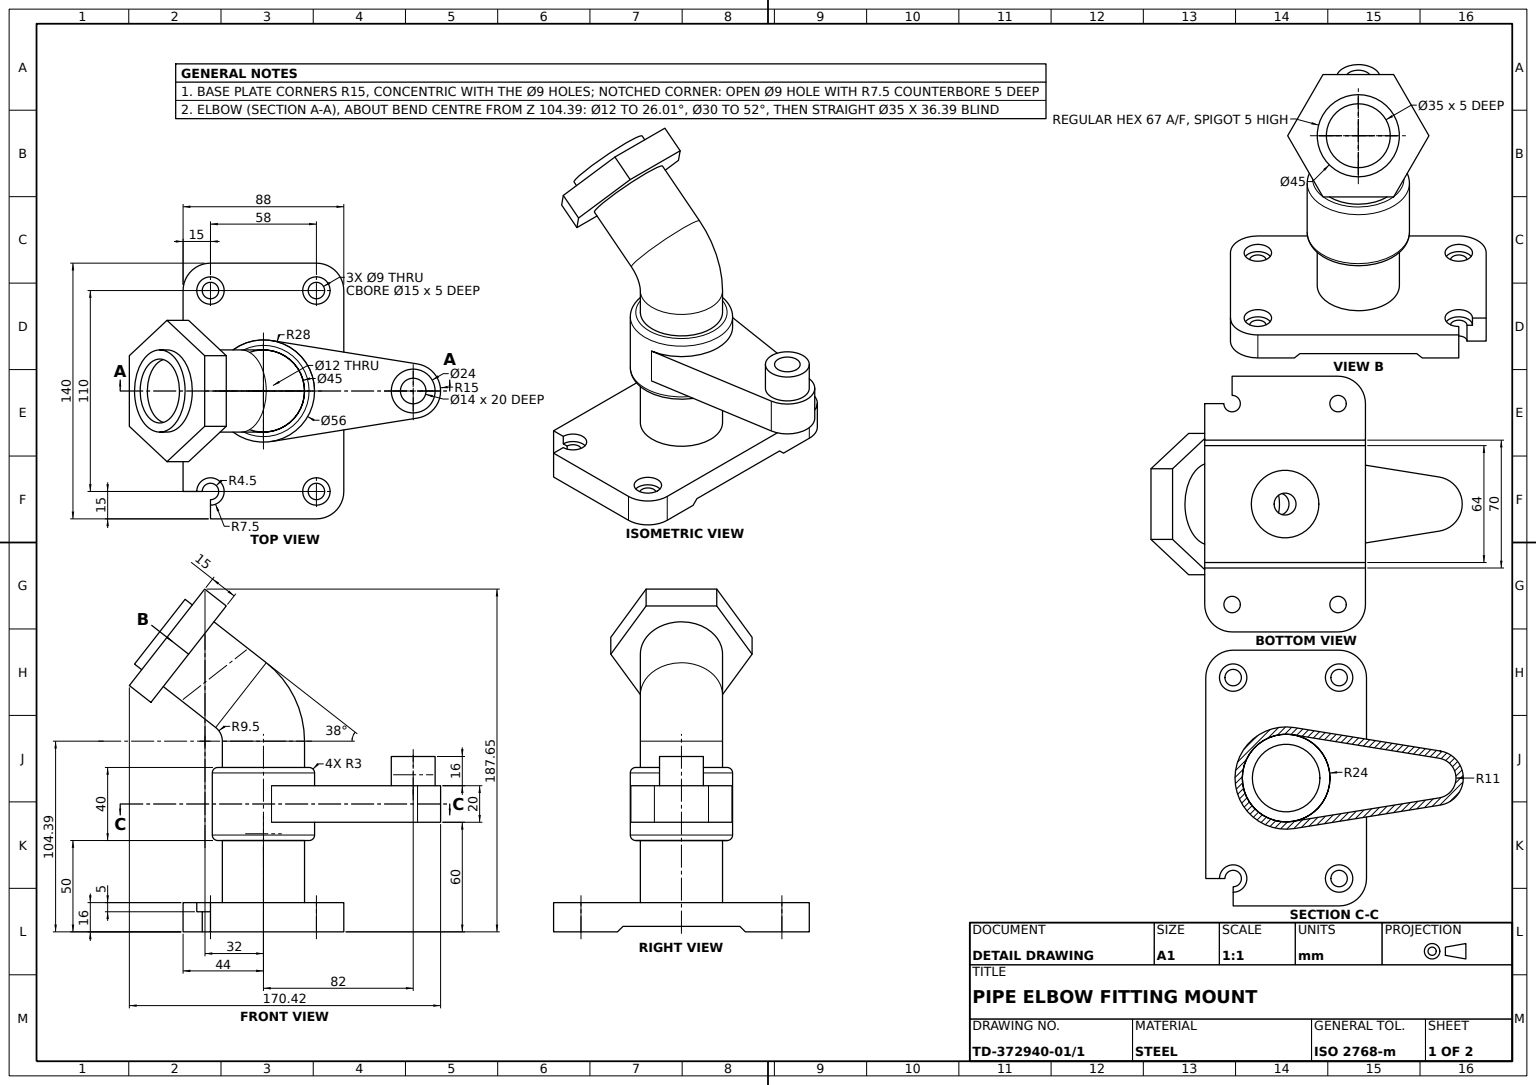
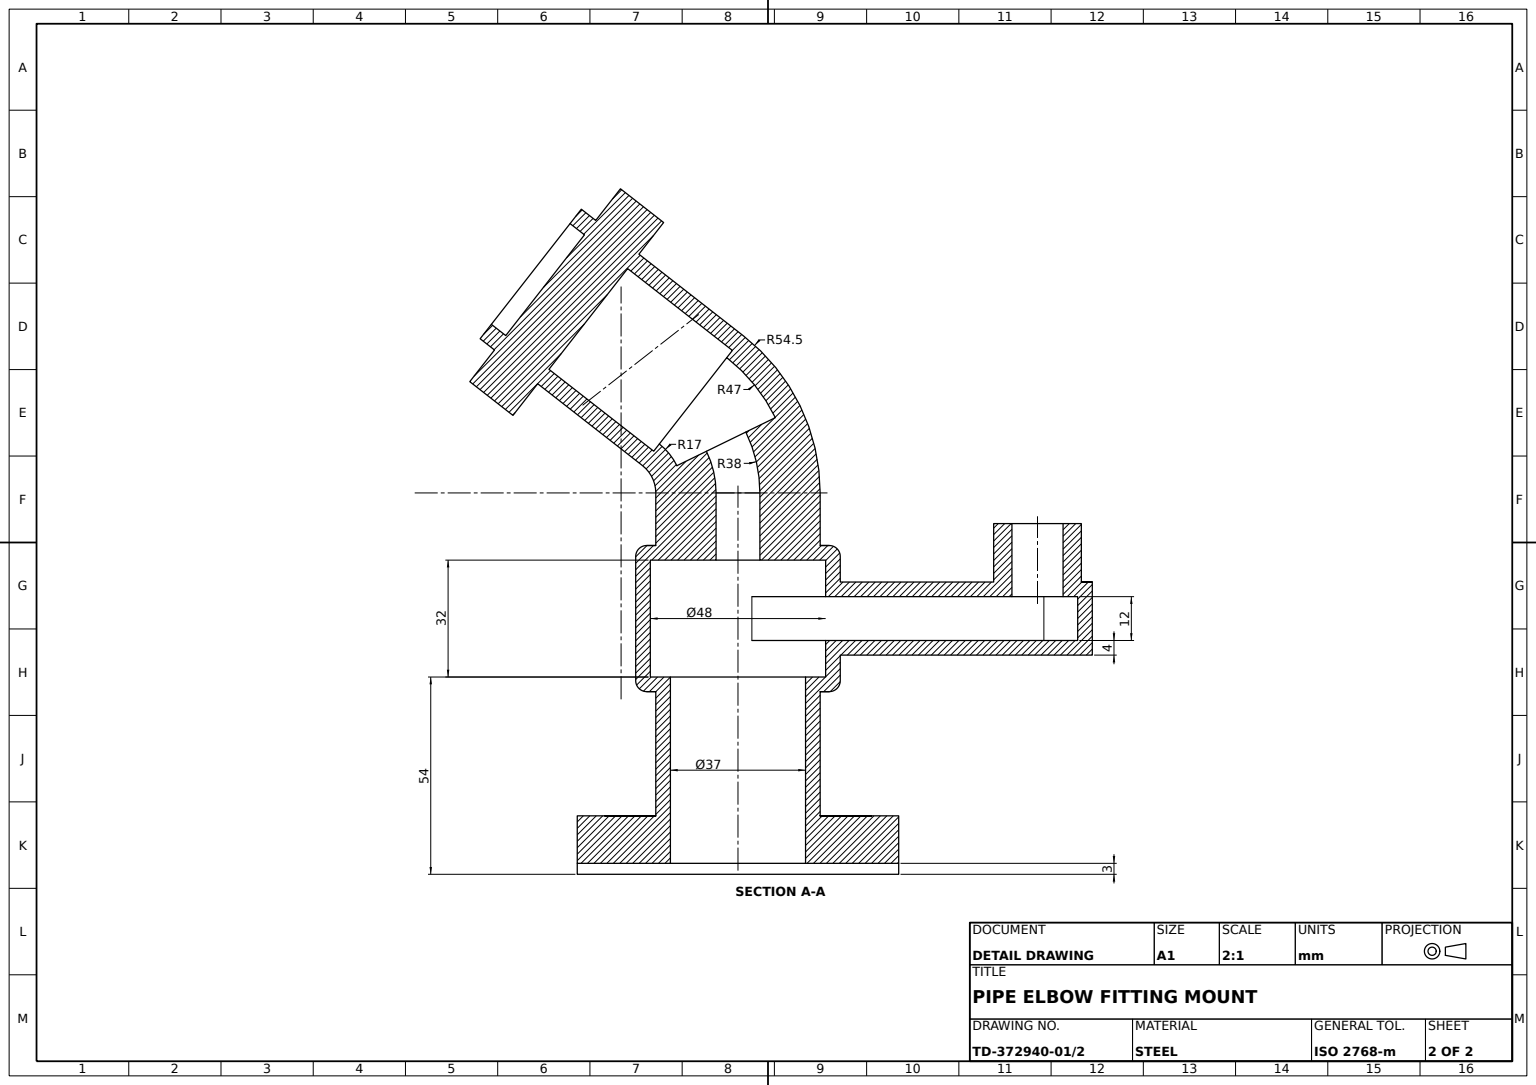
solid
v1 (23.696474,64,-3.804878)
v2 (10.860884,64,-83.743902)
e1 v1 v2 LINE
v3 (-10.860884,64,-83.743902)
e2 v2 v3 CIRCLE(AX(P(0,64,-82),D(0,1,0),D(0,0,1)),11)
v4 (-23.696474,64,-3.804878)
e3 v3 v4 LINE
v5 (0,64,-24)
e4 v4 v5 CIRCLE(AX(P(0,64,0),D(0,-1,0),D(0,0,1)),24)
e5 v5 v1 CIRCLE(AX(P(0,64,0),D(0,-1,0),D(0,0,1)),24)
face PLANE(AX(P(0,64,-82),D(0,1,0),D(0,0,1))) [e1 e2 e3 e4 e5]
v6 (10.860884,76,-83.743902)
v7 (-10.860884,76,-83.743902)
e6 v6 v7 CIRCLE(AX(P(0,76,-82),D(0,1,0),D(0,0,1)),11)
e7 v3 v7 LINE
e8 v2 v6 LINE
face CYL(AX(P(0,64,-82),D(0,1,0),D(0,0,1)),11) rev [e6 -e7 -e2 e8]
v8 (0,178.117814,45.962698)
v9 (0,150.537438,67.51085)
e9 v8 v9 CIRCLE(AX(P(0,164.327626,56.736774),D(0,0.615661475,0.788010754),D(0,-0.788010754,0.615661475)),17.5)
v10 (0,147.459131,63.570796)
e10 v10 v9 LINE
v11 (0,175.039507,42.022645)
e11 v10 v11 CIRCLE(AX(P(0,161.249319,52.79672),D(0,-0.615661475,-0.788010754),D(0,-0.788010754,0.615661475)),17.5)
e12 v11 v8 LINE
face CYL(AX(P(0,129.608901,12.298833),D(0,0.615661475,0.788010754),D(0,-0.788010754,0.615661475)),17.5) rev [e9 -e10 e11 e12]
v12 (-70,0,-29)
v13 (-55,0,-44)
e13 v12 v13 CIRCLE(AX(P(-55,0,-29),D(0,-1,0),D(0,0,1)),15)
v14 (-70,16,-29)
e14 v14 v12 LINE
v15 (-55,16,-44)
e15 v15 v14 CIRCLE(AX(P(-55,16,-29),D(0,1,0),D(0,0,1)),15)
e16 v13 v15 LINE
face CYL(AX(P(-55,16,-29),D(0,-1,0),D(0,0,-1)),15) [-e13 -e14 -e15 -e16]
v16 (55,11,33.5)
v17 (55,11,36.5)
e17 v16 v17 LINE
v18 (59.5,11,29)
e18 v18 v16 CIRCLE(AX(P(55,11,29),D(0,1,0),D(0,0,1)),4.5)
v19 (62.5,11,29)
e19 v18 v19 LINE
e20 v19 v17 CIRCLE(AX(P(55,11,29),D(0,1,0),D(0,0,1)),7.5)
face PLANE(AX(P(59.5,11,29),D(0,-1,0),D(0,0,-1))) rev [-e17 -e18 e19 e20]
v20 (-70,16,29)
e21 v14 v20 LINE
v21 (-70,0,29)
e22 v12 v21 LINE
e23 v21 v20 LINE
face PLANE(AX(P(-70,16,-44),D(1,0,0),D(0,0,-1))) rev [-e21 e14 e22 e23]
v22 (0,146.597384,70.589157)
v23 (0,182.057868,42.884391)
e24 v22 v23 CIRCLE(AX(P(0,164.327626,56.736774),D(0,-0.615661475,-0.788010754),D(0,0.788010754,-0.615661475)),22.5)
e25 v23 v22 CIRCLE(AX(P(0,164.327626,56.736774),D(0,-0.615661475,-0.788010754),D(0,0.788010754,-0.615661475)),22.5)
e26 v9 v8 CIRCLE(AX(P(0,164.327626,56.736774),D(0,0.615661475,0.788010754),D(0,-0.788010754,0.615661475)),17.5)
face PLANE(AX(P(0,164.327626,56.736774),D(0,-0.615661475,-0.788010754),D(0,0.788010754,-0.615661475))) rev [-e24 -e25] [-e26 -e9]
v24 (0,54,18.5)
v25 (0,54,-18.5)
e27 v24 v25 CIRCLE(AX(P(0,54,0),D(0,-1,0),D(0,0,1)),18.5)
e28 v25 v24 CIRCLE(AX(P(0,54,0),D(0,-1,0),D(0,0,1)),18.5)
v26 (0,54,-24)
v27 (0,54,24)
e29 v26 v27 CIRCLE(AX(P(0,54,0),D(0,-1,0),D(0,0,-1)),24)
e30 v27 v26 CIRCLE(AX(P(0,54,0),D(0,-1,0),D(0,0,-1)),24)
face PLANE(AX(P(0,54,24),D(0,1,0),D(0,0,1))) [e27 e28] [-e29 -e30]
v28 (0,80,-97)
v29 (0,60,-97)
e31 v28 v29 LINE
v30 (14.810297,80,-84.378049)
e32 v30 v28 CIRCLE(AX(P(0,80,-82),D(0,1,0),D(0,0,1)),15)
v31 (14.810297,60,-84.378049)
e33 v30 v31 LINE
e34 v31 v29 CIRCLE(AX(P(0,60,-82),D(0,1,0),D(0,0,1)),15)
face CYL(AX(P(0,80,-82),D(0,-1,0),D(0,0,-1)),15) [-e31 -e32 e33 e34]
v32 (0,141.429063,3.063911)
v33 (0,117.78874,21.533755)
e35 v32 v33 CIRCLE(AX(P(0,129.608901,12.298833),D(0,-0.615661475,-0.788010754),D(0,-0.788010754,0.615661475)),15)
v34 (0,125.002777,-10.240014)
e36 v34 v32 CIRCLE(AX(P(0,104.392557,32),D(1,0,0),D(0,0,-1)),47)
v35 (0,111.847318,16.721697)
e37 v35 v34 CIRCLE(AX(P(0,118.425048,3.240841),D(0,0.898723712,0.438515324),D(0,-0.438515324,0.898723712)),15)
e38 v35 v33 CIRCLE(AX(P(0,104.392557,32),D(1,0,0),D(0,0,-1)),17)
face TORUS(AX(P(0,104.392557,32),D(1,0,0),D(0,0,-1)),32,15) rev [-e35 -e36 -e37 e38]
v36 (-55,0,24.5)
v37 (-55,11,24.5)
e39 v36 v37 LINE
v38 (-55,11,33.5)
e40 v37 v38 CIRCLE(AX(P(-55,11,29),D(0,1,0),D(0,0,1)),4.5)
v39 (-55,0,33.5)
e41 v39 v38 LINE
e42 v36 v39 CIRCLE(AX(P(-55,0,29),D(0,1,0),D(0,0,1)),4.5)
face CYL(AX(P(-55,16,29),D(0,1,0),D(0,0,1)),4.5) rev [e39 e40 -e41 -e42]
e43 v33 v32 CIRCLE(AX(P(0,129.608901,12.298833),D(0,-0.615661475,-0.788010754),D(0,-0.788010754,0.615661475)),15)
e44 v34 v35 CIRCLE(AX(P(0,118.425048,3.240841),D(0,0.898723712,0.438515324),D(0,-0.438515324,0.898723712)),15)
face TORUS(AX(P(0,104.392557,32),D(1,0,0),D(0,0,-1)),32,15) rev [-e43 -e38 -e44 e36]
v40 (0,90,-22.5)
v41 (0,104.392557,-22.5)
e45 v40 v41 LINE
v42 (0,104.392557,22.5)
e46 v41 v42 CIRCLE(AX(P(0,104.392557,0),D(0,-1,0),D(0,0,-1)),22.5)
v43 (0,90,22.5)
e47 v43 v42 LINE
e48 v43 v40 CIRCLE(AX(P(0,90,0),D(0,1,0),D(0,0,1)),22.5)
face CYL(AX(P(0,0,0),D(0,1,0),D(0,0,1)),22.5) [e45 e46 -e47 e48]
v44 (0,3,-18.5)
v45 (0,3,18.5)
e49 v44 v45 CIRCLE(AX(P(0,3,0),D(0,1,0),D(0,0,1)),18.5)
e50 v45 v44 CIRCLE(AX(P(0,3,0),D(0,1,0),D(0,0,1)),18.5)
v46 (32,3,-44)
v47 (32,3,44)
e51 v46 v47 LINE
v48 (-32,3,44)
e52 v47 v48 LINE
v49 (-32,3,-44)
e53 v49 v48 LINE
e54 v49 v46 LINE
face PLANE(AX(P(32,3,-97.001),D(0,1,0),D(0,0,1))) rev [e49 e50] [e51 e52 -e53 e54]
v50 (62.5,16,29)
v51 (70,16,29)
e55 v50 v51 LINE
e56 v19 v50 LINE
v52 (59.5,0,29)
e57 v52 v18 LINE
v53 (70,0,29)
e58 v53 v52 LINE
e59 v51 v53 LINE
face PLANE(AX(P(55,-0.001,29),D(0,0,1),D(1,0,0))) [-e55 -e56 -e19 -e57 -e58 -e59]
e60 v40 v43 CIRCLE(AX(P(0,90,0),D(0,1,0),D(0,0,1)),22.5)
v54 (0,90,25)
v55 (0,90,-25)
e61 v54 v55 CIRCLE(AX(P(0,90,0),D(0,1,0),D(0,0,1)),25)
e62 v55 v54 CIRCLE(AX(P(0,90,0),D(0,1,0),D(0,0,1)),25)
face PLANE(AX(P(0,90,0),D(0,1,0),D(0,0,1))) [-e60 -e48] [e61 e62]
v56 (0,80,-28)
v57 (-27.645887,80,-4.439024)
e63 v56 v57 CIRCLE(AX(P(0,80,0),D(0,1,0),D(0,0,1)),28)
v58 (-27.645887,60,-4.439024)
e64 v57 v58 LINE
v59 (0,60,-28)
e65 v59 v58 CIRCLE(AX(P(0,60,0),D(0,1,0),D(0,0,1)),28)
v60 (0,53,-28)
e66 v59 v60 LINE
v61 (0,53,28)
e67 v60 v61 CIRCLE(AX(P(0,53,0),D(0,1,0),D(0,0,1)),28)
v62 (0,87,28)
e68 v62 v61 LINE
v63 (0,87,-28)
e69 v62 v63 CIRCLE(AX(P(0,87,0),D(0,-1,0),D(0,0,1)),28)
e70 v63 v56 LINE
face CYL(AX(P(0,90,0),D(0,-1,0),D(0,0,-1)),28) [e63 e64 -e65 e66 e67 -e68 e69 e70]
e71 v39 v36 CIRCLE(AX(P(-55,0,29),D(0,1,0),D(0,0,1)),4.5)
e72 v38 v37 CIRCLE(AX(P(-55,11,29),D(0,1,0),D(0,0,1)),4.5)
face CYL(AX(P(-55,16,29),D(0,1,0),D(0,0,1)),4.5) rev [-e39 -e71 e41 e72]
v64 (19.341234,125.616036,61.601219)
v65 (38.682468,152.014397,40.976559)
e73 v64 v65 LINE
v66 (38.682468,161.249319,52.79672)
e74 v65 v66 LINE
v67 (19.341234,134.850959,73.42138)
e75 v67 v66 LINE
e76 v64 v67 LINE
face PLANE(AX(P(19.341234,125.616036,61.601219),D(0.866025404,-0.394005377,0.307830738),D(0.414114296,0.91022489,0))) [e73 e74 -e75 -e76]
v68 (0,80,-70)
v69 (0,80,-94)
e77 v68 v69 CIRCLE(AX(P(0,80,-82),D(0,1,0),D(0,0,1)),12)
v70 (0,96,-94)
e78 v70 v69 LINE
v71 (0,96,-70)
e79 v71 v70 CIRCLE(AX(P(0,96,-82),D(0,1,0),D(0,0,1)),12)
e80 v71 v68 LINE
face CYL(AX(P(0,96,-82),D(0,-1,0),D(0,0,-1)),12) [e77 -e78 -e79 e80]
e81 v11 v10 CIRCLE(AX(P(0,161.249319,52.79672),D(0,-0.615661475,-0.788010754),D(0,-0.788010754,0.615661475)),17.5)
face CYL(AX(P(0,129.608901,12.298833),D(0,0.615661475,0.788010754),D(0,-0.788010754,0.615661475)),17.5) rev [e81 e10 e26 -e12]
v72 (0,121.056139,-2.151501)
v73 (0,115.793956,8.633183)
e82 v72 v73 CIRCLE(AX(P(0,118.425048,3.240841),D(0,0.898723712,0.438515324),D(0,-0.438515324,0.898723712)),6)
v74 (0,104.392557,6)
e83 v74 v73 CIRCLE(AX(P(0,104.392557,32),D(1,0,0),D(0,0,-1)),26)
v75 (0,104.392557,-6)
e84 v74 v75 CIRCLE(AX(P(0,104.392557,0),D(0,-1,0),D(0,0,-1)),6)
e85 v75 v72 CIRCLE(AX(P(0,104.392557,32),D(1,0,0),D(0,0,-1)),38)
face TORUS(AX(P(0,104.392557,32),D(1,0,0),D(0,0,-1)),32,6) rev [e82 -e83 e84 e85]
v76 (55,0,-33.5)
v77 (55,11,-33.5)
e86 v76 v77 LINE
v78 (55,0,-24.5)
e87 v78 v76 CIRCLE(AX(P(55,0,-29),D(0,1,0),D(0,0,1)),4.5)
v79 (55,11,-24.5)
e88 v78 v79 LINE
e89 v79 v77 CIRCLE(AX(P(55,11,-29),D(0,1,0),D(0,0,1)),4.5)
face CYL(AX(P(55,16,-29),D(0,1,0),D(0,0,1)),4.5) rev [-e86 -e87 e88 e89]
e90 v24 v45 LINE
e91 v25 v44 LINE
face CYL(AX(P(0,182.058868,0),D(0,-1,0),D(0,0,-1)),18.5) rev [-e27 e90 -e49 -e91]
e92 v70 v71 CIRCLE(AX(P(0,96,-82),D(0,1,0),D(0,0,1)),12)
e93 v69 v68 CIRCLE(AX(P(0,80,-82),D(0,1,0),D(0,0,1)),12)
face CYL(AX(P(0,96,-82),D(0,-1,0),D(0,0,-1)),12) [-e80 -e92 e78 e93]
v80 (-55,16,36.5)
v81 (-55,16,21.5)
e94 v80 v81 CIRCLE(AX(P(-55,16,29),D(0,1,0),D(0,0,1)),7.5)
v82 (-55,11,21.5)
e95 v82 v81 LINE
v83 (-55,11,36.5)
e96 v83 v82 CIRCLE(AX(P(-55,11,29),D(0,1,0),D(0,0,1)),7.5)
e97 v83 v80 LINE
face CYL(AX(P(-55,16,29),D(0,1,0),D(0,0,1)),7.5) rev [e94 -e95 -e96 e97]
v84 (0,143.399089,1.524757)
v85 (0,115.818713,23.072909)
e98 v84 v85 CIRCLE(AX(P(0,129.608901,12.298833),D(0,0.615661475,0.788010754),D(0,-0.788010754,0.615661475)),17.5)
e99 v85 v84 CIRCLE(AX(P(0,129.608901,12.298833),D(0,0.615661475,0.788010754),D(0,-0.788010754,0.615661475)),17.5)
face PLANE(AX(P(0,129.608901,12.298833),D(0,0.615661475,0.788010754),D(0,-0.788010754,0.615661475))) [e43 e35] [e98 e99]
v86 (0,96,-89)
v87 (0,96,-75)
e100 v86 v87 CIRCLE(AX(P(0,96,-82),D(0,1,0),D(0,0,1)),7)
v88 (0,76,-75)
e101 v87 v88 LINE
v89 (0,76,-89)
e102 v89 v88 CIRCLE(AX(P(0,76,-82),D(0,1,0),D(0,0,1)),7)
e103 v86 v89 LINE
face CYL(AX(P(0,182.058868,-82),D(0,-1,0),D(0,0,-1)),7) rev [e100 e101 -e102 -e103]
v90 (-19.341234,125.616036,61.601219)
v91 (-19.341234,134.850959,73.42138)
e104 v90 v91 LINE
v92 (-38.682468,161.249319,52.79672)
e105 v92 v91 LINE
v93 (-38.682468,152.014397,40.976559)
e106 v93 v92 LINE
e107 v93 v90 LINE
face PLANE(AX(P(-38.682468,152.014397,40.976559),D(-0.866025404,-0.394005377,0.307830738),D(0.414114296,-0.91022489,0))) [e104 -e105 -e106 e107]
e108 v82 v83 CIRCLE(AX(P(-55,11,29),D(0,1,0),D(0,0,1)),7.5)
e109 v81 v80 CIRCLE(AX(P(-55,16,29),D(0,1,0),D(0,0,1)),7.5)
face CYL(AX(P(-55,16,29),D(0,1,0),D(0,0,1)),7.5) rev [-e108 e95 e109 -e97]
e110 v77 v79 CIRCLE(AX(P(55,11,-29),D(0,1,0),D(0,0,1)),4.5)
e111 v76 v78 CIRCLE(AX(P(55,0,-29),D(0,1,0),D(0,0,1)),4.5)
face CYL(AX(P(55,16,-29),D(0,1,0),D(0,0,1)),4.5) rev [e110 -e88 -e111 e86]
e112 v42 v41 CIRCLE(AX(P(0,104.392557,0),D(0,-1,0),D(0,0,-1)),22.5)
face CYL(AX(P(0,0,0),D(0,1,0),D(0,0,1)),22.5) [e112 -e45 e60 e47]
v94 (27.645887,80,-4.439024)
e113 v30 v94 LINE
v95 (27.645887,60,-4.439024)
e114 v94 v95 LINE
e115 v31 v95 LINE
face PLANE(AX(P(27.645887,80,-4.439024),D(0.987353104,0,-0.158536585),D(-0.158536585,0,-0.987353104))) [-e33 e113 e114 -e115]
v96 (55,11,-21.5)
v97 (55,11,-36.5)
e116 v96 v97 CIRCLE(AX(P(55,11,-29),D(0,1,0),D(0,0,1)),7.5)
e117 v97 v96 CIRCLE(AX(P(55,11,-29),D(0,1,0),D(0,0,1)),7.5)
face PLANE(AX(P(59.5,11,-29),D(0,-1,0),D(0,0,-1))) rev [-e110 -e89] [e116 e117]
v98 (0,50,25)
v99 (0,50,-25)
e118 v98 v99 CIRCLE(AX(P(0,50,0),D(0,-1,0),D(0,0,1)),25)
e119 v99 v98 CIRCLE(AX(P(0,50,0),D(0,-1,0),D(0,0,1)),25)
v100 (0,50,-22.5)
v101 (0,50,22.5)
e120 v100 v101 CIRCLE(AX(P(0,50,0),D(0,1,0),D(0,0,1)),22.5)
e121 v101 v100 CIRCLE(AX(P(0,50,0),D(0,1,0),D(0,0,1)),22.5)
face PLANE(AX(P(0,50,0),D(0,1,0),D(0,0,1))) rev [e118 e119] [e120 e121]
v102 (0,16,22.5)
e122 v102 v101 LINE
v103 (0,16,-22.5)
e123 v103 v100 LINE
e124 v102 v103 CIRCLE(AX(P(0,16,0),D(0,-1,0),D(0,0,1)),22.5)
face CYL(AX(P(0,0,0),D(0,1,0),D(0,0,1)),22.5) [e122 -e120 -e123 -e124]
v104 (0,86,-24)
v105 (0,86,24)
e125 v104 v105 CIRCLE(AX(P(0,86,0),D(0,-1,0),D(0,0,-1)),24)
e126 v105 v104 CIRCLE(AX(P(0,86,0),D(0,-1,0),D(0,0,-1)),24)
v106 (0,86,6)
v107 (0,86,-6)
e127 v106 v107 CIRCLE(AX(P(0,86,0),D(0,-1,0),D(0,0,-1)),6)
e128 v107 v106 CIRCLE(AX(P(0,86,0),D(0,-1,0),D(0,0,-1)),6)
face PLANE(AX(P(0,86,0),D(0,-1,0),D(0,0,-1))) [e125 e126] [-e127 -e128]
v108 (0,165.804585,30.202483)
v109 (0,138.224209,51.750635)
e129 v108 v109 CIRCLE(AX(P(0,152.014397,40.976559),D(0,-0.615661475,-0.788010754),D(0,-0.788010754,0.615661475)),17.5)
e130 v84 v108 LINE
e131 v85 v109 LINE
face CYL(AX(P(0,129.608901,12.298833),D(0,0.615661475,0.788010754),D(0,-0.788010754,0.615661475)),17.5) rev [-e129 -e130 -e99 e131]
v110 (-14.810297,60,-84.378049)
e132 v110 v58 LINE
e133 v29 v110 CIRCLE(AX(P(0,60,-82),D(0,1,0),D(0,0,1)),15)
e134 v95 v59 CIRCLE(AX(P(0,60,0),D(0,1,0),D(0,0,1)),28)
face PLANE(AX(P(0,60,0),D(0,1,0),D(0,0,1))) rev [e65 -e132 -e133 -e34 e115 e134]
v111 (55,0,44)
v112 (55,16,44)
e135 v111 v112 LINE
v113 (-55,16,44)
e136 v113 v112 LINE
v114 (-55,0,44)
e137 v113 v114 LINE
v115 (-35,0,44)
e138 v114 v115 LINE
e139 v48 v115 LINE
v116 (35,0,44)
e140 v116 v47 LINE
e141 v116 v111 LINE
face PLANE(AX(P(-70,16,44),D(0,0,-1),D(-1,0,0))) rev [e135 -e136 e137 e138 -e139 -e52 -e140 e141]
v117 (55,0,33.5)
e142 v111 v117 LINE
e143 v117 v16 LINE
v118 (55,16,36.5)
e144 v17 v118 LINE
e145 v118 v112 LINE
face PLANE(AX(P(55,-0.001,29),D(-1,0,0),D(0,0,1))) rev [e142 e143 e17 e144 e145 -e135]
v119 (23.696474,76,-3.804878)
e146 v1 v119 LINE
e147 v119 v6 LINE
face PLANE(AX(P(23.696474,64,-3.804878),D(0.987353104,0,-0.158536585),D(-0.158536585,0,-0.987353104))) rev [e146 e147 -e8 -e1]
v120 (0,134.284155,54.828942)
v121 (0,169.744639,27.124176)
e148 v120 v121 CIRCLE(AX(P(0,152.014397,40.976559),D(0,0.615661475,0.788010754),D(0,-0.788010754,0.615661475)),22.5)
e149 v121 v120 CIRCLE(AX(P(0,152.014397,40.976559),D(0,0.615661475,0.788010754),D(0,-0.788010754,0.615661475)),22.5)
v122 (-19.341234,178.412757,20.3519)
e150 v122 v93 LINE
v123 (19.341234,178.412757,20.3519)
e151 v123 v122 LINE
e152 v65 v123 LINE
e153 v90 v64 LINE
face PLANE(AX(P(0,77.499083,99.194303),D(0,0.615661475,0.788010754),D(0,-0.788010754,0.615661475))) rev [e148 e149] [-e150 -e151 -e152 -e73 -e153 -e107]
v124 (0,147.339143,-1.55355)
e154 v124 v121 LINE
v125 (0,111.878659,26.151216)
e155 v125 v124 CIRCLE(AX(P(0,129.608901,12.298833),D(0,-0.615661475,-0.788010754),D(0,0.788010754,-0.615661475)),22.5)
e156 v125 v120 LINE
face CYL(AX(P(0,129.608901,12.298833),D(0,0.615661475,0.788010754),D(0,-0.788010754,0.615661475)),22.5) [-e154 -e155 e156 -e149]
e157 v106 v74 LINE
e158 v107 v75 LINE
face CYL(AX(P(0,-5,0),D(0,1,0),D(0,0,1)),6) rev [-e84 -e157 e127 e158]
e159 v62 v54 CIRCLE(AX(P(0,87,25),D(-1,0,0),D(0,0,1)),3)
e160 v63 v55 CIRCLE(AX(P(0,87,-25),D(1,0,0),D(0,0,-1)),3)
face TORUS(AX(P(0,87,0),D(0,1,0),D(0,0,1)),25,3) [e159 -e62 -e160 -e69]
e161 v103 v102 CIRCLE(AX(P(0,16,0),D(0,-1,0),D(0,0,1)),22.5)
face CYL(AX(P(0,0,0),D(0,1,0),D(0,0,1)),22.5) [e123 -e121 -e122 -e161]
e162 v105 v27 LINE
v126 (0,76,-24)
e163 v104 v126 LINE
e164 v126 v119 CIRCLE(AX(P(0,76,0),D(0,-1,0),D(0,0,1)),24)
e165 v5 v26 LINE
face CYL(AX(P(0,0,0),D(0,-1,0),D(0,0,-1)),24) rev [-e162 -e125 e163 e164 -e146 -e5 e165 e29]
v127 (35,0,-44)
e166 v127 v116 LINE
v128 (55,0,-44)
e167 v128 v127 LINE
v129 (70,0,-29)
e168 v128 v129 CIRCLE(AX(P(55,0,-29),D(0,-1,0),D(0,0,1)),15)
e169 v53 v129 LINE
e170 v52 v117 CIRCLE(AX(P(55,0,29),D(0,1,0),D(0,0,1)),4.5)
face PLANE(AX(P(0,0,0),D(0,1,0),D(0,0,1))) rev [e87 e111] [-e141 -e166 -e167 e168 -e169 e58 e170 -e142]
v130 (-55,0,-24.5)
v131 (-55,11,-24.5)
e171 v130 v131 LINE
v132 (-55,0,-33.5)
e172 v132 v130 CIRCLE(AX(P(-55,0,-29),D(0,1,0),D(0,0,1)),4.5)
v133 (-55,11,-33.5)
e173 v132 v133 LINE
e174 v133 v131 CIRCLE(AX(P(-55,11,-29),D(0,1,0),D(0,0,1)),4.5)
face CYL(AX(P(-55,16,-29),D(0,1,0),D(0,0,1)),4.5) rev [-e171 -e172 e173 e174]
v134 (-55,16,-21.5)
v135 (-55,16,-36.5)
e175 v134 v135 CIRCLE(AX(P(-55,16,-29),D(0,1,0),D(0,0,1)),7.5)
e176 v135 v134 CIRCLE(AX(P(-55,16,-29),D(0,1,0),D(0,0,1)),7.5)
e177 v50 v118 CIRCLE(AX(P(55,16,29),D(0,1,0),D(0,0,1)),7.5)
v136 (70,16,-29)
e178 v51 v136 LINE
v137 (55,16,-44)
e179 v136 v137 CIRCLE(AX(P(55,16,-29),D(0,1,0),D(0,0,1)),15)
e180 v137 v15 LINE
e181 v20 v113 CIRCLE(AX(P(-55,16,29),D(0,1,0),D(0,0,1)),15)
v138 (55,16,-36.5)
v139 (55,16,-21.5)
e182 v138 v139 CIRCLE(AX(P(55,16,-29),D(0,1,0),D(0,0,1)),7.5)
e183 v139 v138 CIRCLE(AX(P(55,16,-29),D(0,1,0),D(0,0,1)),7.5)
face PLANE(AX(P(0,16,0),D(0,1,0),D(0,0,1))) [-e109 -e94] [-e175 -e176] [-e177 e55 e178 e179 e180 e15 e21 e181 e136 -e145] [e161 e124] [-e182 -e183]
v140 (-55,11,-21.5)
e184 v140 v134 LINE
v141 (-55,11,-36.5)
e185 v141 v135 LINE
e186 v140 v141 CIRCLE(AX(P(-55,11,-29),D(0,1,0),D(0,0,1)),7.5)
face CYL(AX(P(-55,16,-29),D(0,1,0),D(0,0,1)),7.5) rev [e184 e175 -e185 -e186]
e187 v129 v136 LINE
face PLANE(AX(P(70,16,-44),D(-1,0,0),D(0,0,1))) rev [e169 e187 -e178 e59]
e188 v94 v56 CIRCLE(AX(P(0,80,0),D(0,1,0),D(0,0,1)),28)
e189 v63 v62 CIRCLE(AX(P(0,87,0),D(0,-1,0),D(0,0,1)),28)
e190 v61 v60 CIRCLE(AX(P(0,53,0),D(0,1,0),D(0,0,1)),28)
face CYL(AX(P(0,90,0),D(0,-1,0),D(0,0,-1)),28) [-e114 e188 -e70 e189 e68 e190 -e66 -e134]
e191 v137 v128 LINE
face CYL(AX(P(55,16,-29),D(0,-1,0),D(0,0,-1)),15) [-e168 -e191 -e179 -e187]
e192 v141 v140 CIRCLE(AX(P(-55,11,-29),D(0,1,0),D(0,0,1)),7.5)
face CYL(AX(P(-55,16,-29),D(0,1,0),D(0,0,1)),7.5) rev [-e192 e185 e176 -e184]
e193 v98 v61 CIRCLE(AX(P(0,53,25),D(-1,0,0),D(0,0,1)),3)
e194 v99 v60 CIRCLE(AX(P(0,53,-25),D(1,0,0),D(0,0,-1)),3)
face TORUS(AX(P(0,53,0),D(0,1,0),D(0,0,1)),25,3) [e193 -e67 -e194 -e118]
v142 (-23.696474,76,-3.804878)
e195 v4 v142 LINE
e196 v142 v126 CIRCLE(AX(P(0,76,0),D(0,-1,0),D(0,0,1)),24)
face CYL(AX(P(0,0,0),D(0,-1,0),D(0,0,-1)),24) rev [e30 -e165 -e4 e195 e196 -e163 -e126 e162]
v143 (0,143.519077,66.649104)
e197 v143 v22 LINE
v144 (0,178.979561,38.944337)
e198 v144 v23 LINE
e199 v144 v143 CIRCLE(AX(P(0,161.249319,52.79672),D(0,0.615661475,0.788010754),D(0,-0.788010754,0.615661475)),22.5)
face CYL(AX(P(0,129.608901,12.298833),D(0,0.615661475,0.788010754),D(0,-0.788010754,0.615661475)),22.5) [e197 e24 -e198 e199]
v145 (-35,0,-44)
e200 v145 v115 LINE
e201 v145 v49 LINE
face PLANE(AX(P(-35,0,-97.001),D(-0.707106781,0.707106781,0),D(-0.707106781,-0.707106781,0))) rev [e53 e139 -e200 e201]
face CYL(AX(P(55,16,29),D(0,1,0),D(0,0,1)),4.5) rev [-e143 -e170 e57 e18]
e202 v114 v21 CIRCLE(AX(P(-55,0,29),D(0,-1,0),D(0,0,1)),15)
e203 v145 v13 LINE
e204 v130 v132 CIRCLE(AX(P(-55,0,-29),D(0,1,0),D(0,0,1)),4.5)
face PLANE(AX(P(0,0,0),D(0,1,0),D(0,0,1))) rev [e42 e71] [-e138 e202 -e22 e13 -e203 e200] [e172 e204]
v146 (-19.341234,187.647679,32.172061)
e205 v122 v146 LINE
v147 (19.341234,187.647679,32.172061)
e206 v147 v146 LINE
e207 v123 v147 LINE
face PLANE(AX(P(19.341234,178.412757,20.3519),D(0,0.788010754,-0.615661475),D(0,0.615661475,0.788010754))) [e151 e205 -e206 -e207]
v148 (-14.810297,80,-84.378049)
e208 v148 v57 LINE
e209 v148 v110 LINE
face PLANE(AX(P(-27.645887,80,-4.439024),D(0.987353104,0,0.158536585),D(0.158536585,0,-0.987353104))) rev [e132 -e64 -e208 e209]
e210 v66 v147 LINE
face PLANE(AX(P(38.682468,152.014397,40.976559),D(0.866025404,0.394005377,-0.307830738),D(-0.414114296,0.91022489,0))) [-e74 e152 e207 -e210]
e211 v131 v133 CIRCLE(AX(P(-55,11,-29),D(0,1,0),D(0,0,1)),4.5)
face CYL(AX(P(-55,16,-29),D(0,1,0),D(0,0,1)),4.5) rev [-e173 -e204 e171 e211]
e212 v73 v72 CIRCLE(AX(P(0,118.425048,3.240841),D(0,0.898723712,0.438515324),D(0,-0.438515324,0.898723712)),6)
face PLANE(AX(P(0,118.425048,3.240841),D(0,0.898723712,0.438515324),D(0,-0.438515324,0.898723712))) [e37 e44] [-e212 -e82]
face PLANE(AX(P(-50.5,11,-29),D(0,-1,0),D(0,0,-1))) rev [e192 e186] [-e211 -e174]
face CYL(AX(P(0,182.058868,0),D(0,-1,0),D(0,0,-1)),18.5) rev [-e90 -e28 e91 -e50]
e213 v75 v74 CIRCLE(AX(P(0,104.392557,0),D(0,-1,0),D(0,0,-1)),6)
face TORUS(AX(P(0,104.392557,32),D(1,0,0),D(0,0,-1)),32,6) rev [e213 e83 e212 -e85]
e214 v146 v92 LINE
face PLANE(AX(P(-19.341234,178.412757,20.3519),D(-0.866025404,0.394005377,-0.307830738),D(-0.414114296,-0.91022489,0))) [e150 e106 -e214 -e205]
face CYL(AX(P(0,-5,0),D(0,1,0),D(0,0,1)),6) rev [e128 e157 -e213 -e158]
e215 v7 v142 LINE
face PLANE(AX(P(-10.860884,64,-83.743902),D(-0.987353104,0,-0.158536585),D(-0.158536585,0,0.987353104))) rev [-e3 e7 e215 -e195]
face PLANE(AX(P(0,86.734005,111.014464),D(0,0.615661475,0.788010754),D(0,-0.788010754,0.615661475))) [-e81 -e11]
e216 v91 v67 LINE
e217 v143 v144 CIRCLE(AX(P(0,161.249319,52.79672),D(0,0.615661475,0.788010754),D(0,-0.788010754,0.615661475)),22.5)
face PLANE(AX(P(0,86.734005,111.014464),D(0,0.615661475,0.788010754),D(0,-0.788010754,0.615661475))) [e105 e216 e75 e210 e206 e214] [-e217 -e199]
e218 v124 v125 CIRCLE(AX(P(0,129.608901,12.298833),D(0,-0.615661475,-0.788010754),D(0,0.788010754,-0.615661475)),22.5)
face CYL(AX(P(0,129.608901,12.298833),D(0,0.615661475,0.788010754),D(0,-0.788010754,0.615661475)),22.5) [-e148 -e156 -e218 e154]
e219 v46 v127 LINE
face PLANE(AX(P(-70,16,-44),D(0,0,1),D(1,0,0))) rev [e167 -e219 -e54 -e201 e203 e16 -e180 e191]
e220 v41 v124 CIRCLE(AX(P(0,104.392557,32),D(1,0,0),D(0,0,-1)),54.5)
e221 v42 v125 CIRCLE(AX(P(0,104.392557,32),D(1,0,0),D(0,0,-1)),9.5)
face TORUS(AX(P(0,104.392557,32),D(1,0,0),D(0,0,-1)),32,22.5) [e155 -e220 -e112 e221]
face PLANE(AX(P(35,0,-97.001),D(0.707106781,0.707106781,0),D(-0.707106781,0.707106781,0))) rev [-e51 e219 e166 e140]
e222 v87 v86 CIRCLE(AX(P(0,96,-82),D(0,1,0),D(0,0,1)),7)
face PLANE(AX(P(0,96,-82),D(0,1,0),D(0,0,1))) [-e100 -e222] [e79 e92]
e223 v109 v108 CIRCLE(AX(P(0,152.014397,40.976559),D(0,-0.615661475,-0.788010754),D(0,-0.788010754,0.615661475)),17.5)
face CYL(AX(P(0,129.608901,12.298833),D(0,0.615661475,0.788010754),D(0,-0.788010754,0.615661475)),17.5) rev [-e98 e130 -e223 -e131]
face TORUS(AX(P(0,104.392557,32),D(1,0,0),D(0,0,-1)),32,22.5) [e218 -e221 -e46 e220]
e224 v88 v89 CIRCLE(AX(P(0,76,-82),D(0,1,0),D(0,0,1)),7)
face CYL(AX(P(0,182.058868,-82),D(0,-1,0),D(0,0,-1)),7) rev [e103 -e224 -e101 e222]
face CYL(AX(P(0,129.608901,12.298833),D(0,0.615661475,0.788010754),D(0,-0.788010754,0.615661475)),22.5) [e198 e25 -e197 e217]
face PLANE(AX(P(-50.5,11,29),D(0,-1,0),D(0,0,-1))) rev [-e40 -e72] [e96 e108]
face TORUS(AX(P(0,53,0),D(0,1,0),D(0,0,1)),25,3) [-e119 e194 -e190 -e193]
face CYL(AX(P(-55,16,29),D(0,-1,0),D(0,0,-1)),15) [-e23 -e202 -e137 -e181]
face TORUS(AX(P(0,87,0),D(0,1,0),D(0,0,1)),25,3) [-e159 -e189 e160 -e61]
face PLANE(AX(P(-19.341234,125.616036,61.601219),D(0,-0.788010754,0.615661475),D(0,-0.615661475,-0.788010754))) [-e104 e153 e76 -e216]
face PLANE(AX(P(0,77.499083,99.194303),D(0,0.615661475,0.788010754),D(0,-0.788010754,0.615661475))) rev [e129 e223]
e225 v28 v148 CIRCLE(AX(P(0,80,-82),D(0,1,0),D(0,0,1)),15)
face CYL(AX(P(0,80,-82),D(0,-1,0),D(0,0,-1)),15) [-e225 e31 e133 -e209]
face PLANE(AX(P(0,76,-82),D(0,1,0),D(0,0,1))) rev [-e164 -e196 -e215 -e6 -e147] [e102 e224]
e226 v96 v139 LINE
e227 v97 v138 LINE
face CYL(AX(P(55,16,-29),D(0,1,0),D(0,0,1)),7.5) rev [e182 -e226 -e117 e227]
face CYL(AX(P(55,16,-29),D(0,1,0),D(0,0,1)),7.5) rev [e183 -e227 -e116 e226]
face PLANE(AX(P(0,80,0),D(0,1,0),D(0,0,1))) [-e77 -e93] [e208 -e63 -e188 -e113 e32 e225]
face CYL(AX(P(55,16,29),D(0,1,0),D(0,0,1)),7.5) rev [-e144 -e20 e56 e177]
